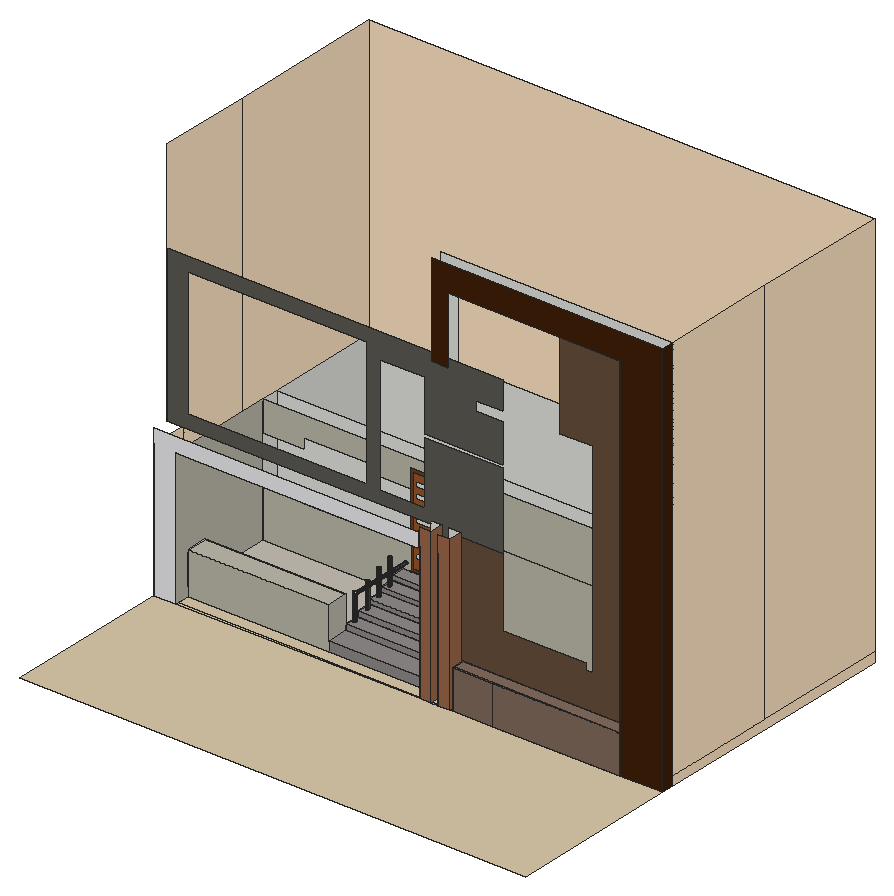
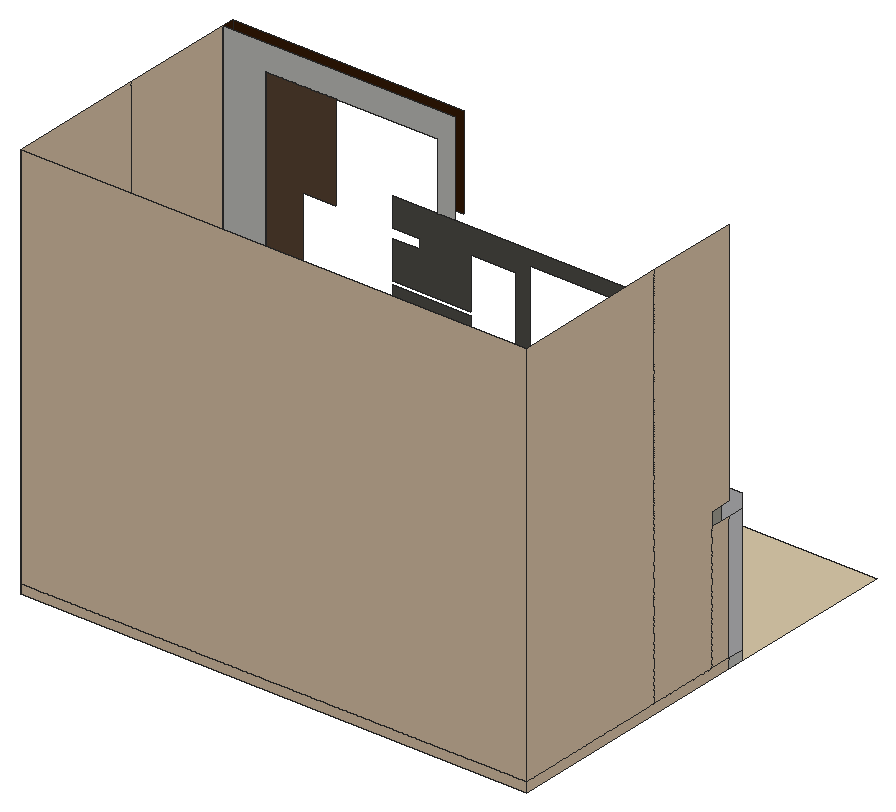
# SketchUp Ruby script. Lengths in inches.
U = 1.inch
M = Sketchup.active_model
def pt(a) = Geom::Point3d.new(a.map { |v| v * U })
def face(e, loops, mat)
  f = e.add_face(loops[0].map { |a| pt(a) })
  loops[1..].each { |l| e.add_face(l.map { |a| pt(a) }).erase! }
  f.material = f.back_material = mat if mat
  f
end
# faces: each face lists its corners as indices into pts; further lists are holes
def faces(e, pts, list, mat = nil) = list.each { |f| face(e, (f[0].is_a?(Array) ? f : [f]).map { |l| l.map { |i| pts[i] } }, mat) }
# xy, xz, yz: faces in a plane at the given z, y or x. An outline is a flat list of corners, or four numbers for a rectangle; further outlines are holes
def ring(l) = l.size == 4 ? [[l[0], l[1]], [l[2], l[1]], [l[2], l[3]], [l[0], l[3]]] : l.each_slice(2).to_a
def flat(e, list, mat, &to3) = list.each { |f| face(e, (f[0].is_a?(Array) ? f : [f]).map { |l| ring(l).map { |u, v| to3.(u, v) } }, mat) }
def xy(e, z, list, mat = nil) = flat(e, list, mat) { |x, y| [x, y, z] }
def xz(e, y, list, mat = nil) = flat(e, list, mat) { |x, z| [x, y, z] }
def yz(e, x, list, mat = nil) = flat(e, list, mat) { |y, z| [x, y, z] }
def lines(e, pts, list) = list.each { |a, b| e.add_line(pt(pts[a]), pt(pts[b])) }
# prism: a flat outline (further loops are holes) pulled along v
def prism(e, loops, v, mat = nil)
  f = face(e, loops, mat); d = Geom::Vector3d.new(v.map { |x| x * U })
  f.pushpull(f.normal.samedirection?(d) ? d.length : -d.length)
end
def box(e, o, s, mat = nil) = prism(e, [[o, [o[0] + s[0], o[1], o[2]], [o[0] + s[0], o[1] + s[1], o[2]], [o[0], o[1] + s[1], o[2]]]], [0, 0, s[2]], mat)
def at(x, y, z, deg = 0) = Geom::Transformation.translation(pt([x, y, z])) * Geom::Transformation.rotation(ORIGIN, Z_AXIS, deg.degrees)
def axes(o, x, y, z) = Geom::Transformation.new([*x, 0, *y, 0, *z, 0, *pt(o).to_a, 1])
def part(name) = M.definitions.add(name)
# library, detail: a bought-in or finely detailed component or shape, given as its bounding box
def library(name, o, s) = part(name).tap { |d| box(d.entities, o, s) }
def detail(e, o, s) = box(e.add_group.entities, o, s)
def put(e, d, t, mat = nil) = e.add_instance(d, t).tap { |i| i.material = mat if mat }
def group(e, t, mat = nil) = e.add_group.tap { |g| g.transformation = t; g.material = mat if mat }.entities
root = M.entities
M.materials.add("[0012_Bisque]").color = [255, 228, 196]
M.materials.add("[0043_SaddleBrown]").color = [63, 31, 8]
M.materials.add("[Blinds Vertical Pattern]").color = [237, 237, 239]
M.materials.add("[Cladding Siding Tan]").color = [102, 79, 59]
M.materials.add("[Field Rectangle Tile]").color = [196, 189, 179]
M.materials.add("[Field Square Tile]").color = [217, 201, 169]
M.materials.add("[Formica Graystone]").color = [91, 89, 83]
M.materials.add("[Formica Graystone]1").color = [188, 184, 170]
M.materials.add("[Granite Brown]").color = [130, 107, 93]
M.materials.add("[Quartz Light Grey]").color = [251, 251, 252]
M.materials.add("[Stone Marble]").color = [143, 138, 136]
M.materials.add("[Wood Cherry Original]").color = [152, 86, 42]
M.materials.add("[Wood Veneer 01]").color = [107, 62, 33]
M.materials.add("[Wood Veneer 01]1").color = [120, 70, 37]
M.materials.add("[Wood Veneer 02]").color = [155, 104, 74]
xy(root,0,[[0,159.45,20.26,162.83],[250.29,161.27,261.4375,162.83],[267.85,161.27,267.85,162.83,279,162.83,279,161.35],[267.85,161.27,279,161.35,279,161.27],[0,162.83,20.26,174.45],
  [250.29,162.83,261.4375,174.45],[267.85,162.83,279,174.45],[281.23,162.83,439.49,174.45],[439.49,162.83,480,174.45],[0,174.45,480,414.45]])
xy(root,0,[[0,0,0,159.45,20.26,159.45,250.29,161.14,250.29,161.27,261.4375,161.27,261.4375,161.22,267.85,161.27,279,161.27,279,161.35,319.23,161.65,439.49,162.53,480,162.83,480,0],[20.26,159.45,20.26,162.83,250.29,162.83,250.29,161.14],[261.4375,161.22,261.4375,162.83,267.85,162.83,267.85,161.27],[279,161.35,279,162.83,281.23,162.83,281.23,161.65,319.23,161.65],[20.26,162.83,250.29,174.45],
  [261.4375,162.83,267.85,174.45],[279,162.83,281.23,174.45]],"[Field Square Tile]")
xy(root,0,[[281.23,161.65,281.23,162.83,439.49,162.83,439.49,162.53,319.23,161.65],[439.49,162.53,439.49,162.83,480,162.83]],"[Quartz Light Grey]")
xy(root,9,[[439.49,174.45,459.74,194.72,459.74,283.36,480,283.36,480,174.45],[0,194.72,20.26,263.11],[153.32,194.72,250.29,208.86],[153.32,208.86,250.29,223],[153.32,223,250.29,236.75],
  [153.32,236.75,250.29,249.88],[153.32,249.88,250.29,263.11],[0,263.11,0,414.45,480,414.45,480,283.36,459.74,283.36,459.74,394.19,20.26,394.19,20.26,263.11],[20.26,263.11,459.74,279.66],[20.26,279.66,459.74,394.19]])
xy(root,9,[[20.26,194.72,153.32,263.11],[250.29,194.72,459.74,263.11]],"[Field Rectangle Tile]")
xy(root,9,[[153.32,174.45,250.29,194.72]],"[Stone Marble]")
xy(root,14.375,[[156.2,200.96,155.83,201.01,155.48,201.15,155.18,201.38,154.95,201.68,154.8125,202.03,154.76,202.4,154.8125,202.77,154.95,203.12,155.18,203.41,155.48,203.64,155.83,203.79,156.2,203.84,156.57,203.79,156.92,203.64,157.22,203.41,157.44,203.12,157.59,202.77,157.64,202.4,157.59,202.03,157.44,201.68,157.22,201.38,156.92,201.15,156.57,201.01]])
xy(root,14.375,[[[153.32,194.72,250.29,208.86],[156.2,200.96,155.83,201.01,155.48,201.15,155.18,201.38,154.95,201.68,154.8125,202.03,154.76,202.4,154.8125,202.77,154.95,203.12,155.18,203.41,155.48,203.64,155.83,203.79,156.2,203.84,156.57,203.79,156.92,203.64,157.22,203.41,157.44,203.12,157.59,202.77,157.64,202.4,157.59,202.03,157.44,201.68,157.22,201.38,156.92,201.15,156.57,201.01]]],"[Stone Marble]")
xy(root,19.125,[[157.37,214.23,157,214.28,156.65,214.43,156.35,214.66,156.125,214.95,155.98,215.3,155.93,215.67,155.98,216.04,156.125,216.39,156.35,216.6875,156.65,216.92,157,217.0625,157.37,217.11,157.74,217.0625,158.09,216.92,158.39,216.6875,158.62,216.39,158.76,216.04,158.81,215.67,158.76,215.3,158.62,214.95,158.39,214.66,158.09,214.43,157.74,214.28]])
xy(root,19.125,[[[153.32,208.86,250.29,223],[157.37,214.23,157,214.28,156.65,214.43,156.35,214.66,156.125,214.95,155.98,215.3,155.93,215.67,155.98,216.04,156.125,216.39,156.35,216.6875,156.65,216.92,157,217.0625,157.37,217.11,157.74,217.0625,158.09,216.92,158.39,216.6875,158.62,216.39,158.76,216.04,158.81,215.67,158.76,215.3,158.62,214.95,158.39,214.66,158.09,214.43,157.74,214.28]]],"[Stone Marble]")
xy(root,23.5,[[156.56,228.62,156.1875,228.66,155.84,228.81,155.54,229.04,155.3125,229.33,155.17,229.68,155.12,230.05,155.17,230.43,155.3125,230.77,155.54,231.07,155.84,231.3,156.1875,231.44,156.56,231.49,156.93,231.44,157.28,231.3,157.57,231.07,157.8,230.77,157.95,230.43,158,230.05,157.95,229.68,157.8,229.33,157.57,229.04,157.28,228.81,156.93,228.66]])
xy(root,23.5,[[[153.32,223,250.29,236.75],[156.56,228.62,156.1875,228.66,155.84,228.81,155.54,229.04,155.3125,229.33,155.17,229.68,155.12,230.05,155.17,230.43,155.3125,230.77,155.54,231.07,155.84,231.3,156.1875,231.44,156.56,231.49,156.93,231.44,157.28,231.3,157.57,231.07,157.8,230.77,157.95,230.43,158,230.05,157.95,229.68,157.8,229.33,157.57,229.04,157.28,228.81,156.93,228.66]]],"[Stone Marble]")
xy(root,27.3125,[[157.29,241.24,156.92,241.29,156.57,241.43,156.27,241.66,156.04,241.96,155.9,242.31,155.85,242.68,155.9,243.05,156.04,243.4,156.27,243.7,156.57,243.92,156.92,244.07,157.29,244.12,157.66,244.07,158.01,243.92,158.3,243.7,158.53,243.4,158.68,243.05,158.72,242.68,158.68,242.31,158.53,241.96,158.3,241.66,158.01,241.43,157.66,241.29]])
xy(root,27.3125,[[[153.32,236.75,250.29,249.88],[157.29,241.24,156.92,241.29,156.57,241.43,156.27,241.66,156.04,241.96,155.9,242.31,155.85,242.68,155.9,243.05,156.04,243.4,156.27,243.7,156.57,243.92,156.92,244.07,157.29,244.12,157.66,244.07,158.01,243.92,158.3,243.7,158.53,243.4,158.68,243.05,158.72,242.68,158.68,242.31,158.53,241.96,158.3,241.66,158.01,241.43,157.66,241.29]]],"[Stone Marble]")
xy(root,31.75,[[153.32,249.88,250.29,263.11]],"[Stone Marble]")
xy(root,36.58,[[281.23,161.65,319.23,161.65,439.49,162.53,439.49,162.83,281.23,162.83],[281.23,162.83,439.49,174.45]],"[Granite Brown]")
xy(root,38.75,[[156.2,200.96,155.83,201.01,155.48,201.15,155.18,201.38,154.95,201.68,154.8125,202.03,154.76,202.4,154.8125,202.77,154.95,203.12,155.18,203.41,155.48,203.64,155.83,203.79,156.2,203.84,156.57,203.79,156.92,203.64,157.22,203.41,157.44,203.12,157.59,202.77,157.64,202.4,157.59,202.03,157.44,201.68,157.22,201.38,156.92,201.15,156.57,201.01]])
xy(root,39.75,[[156.2,200.96,156.57,201.01,156.92,201.15,157.22,201.38,157.44,201.68,157.59,202.03,157.64,202.4,157.59,202.77,157.44,203.12,157.22,203.41,156.92,203.64,156.57,203.79,156.2,203.84,155.83,203.79,155.48,203.64,155.18,203.41,154.95,203.12,154.8125,202.77,154.76,202.4,154.8125,202.03,154.95,201.68,155.18,201.38,155.48,201.15,155.83,201.01]])
xy(root,39.75,[[20.26,174.45,153.32,194.72]],"[Formica Graystone]1")
xz(root,159.45,[[0,0,20.26,0,20.26,129,250.29,129,250.29,142.5625,0,142.5625]],"[Blinds Vertical Pattern]")
xz(root,161.27,[[250.29,0,261.4375,145.3125],[267.85,0,279,145.3125]],"[Wood Veneer 02]")
xz(root,161.65,[[281.23,0,319.23,36.58]],"[Granite Brown]")
xz(root,162.83,[[439.49,0,480,0,480,377.375,260.36,377.375,260.36,289.4375,276.43,289.4375,276.43,352.96,439.49,352.96]],"[0043_SaddleBrown]")
xz(root,174.45,[[250.29,0,261.4375,9],[267.85,0,279,9],[281.23,0,439.49,36.58],[439.49,0,480,9],[250.29,9,261.4375,145.3125],
  [439.49,9,439.49,352.96,276.43,352.96,276.43,289.4375,260.36,289.4375,260.36,377.375,480,377.375,480,9],[267.85,9,279,145.3125]])
xz(root,174.45,[[279,0,281.23,0,281.23,36.58,439.49,36.58,439.49,352.96,372.71,352.96,372.71,262.44,404.1,262.44,404.1,69.56,397.29,69.56,397.29,75.51,319.23,75.51,319.23,141.375,279,141.375]],"[Cladding Siding Tan]")
xz(root,174.45,[[261.4375,0,267.85,0,267.85,145.3125,279,145.3125,279,141.375,319.23,141.375,319.23,213.94,244.42,213.94,244.42,154.2,202.17,154.2,202.17,265.33,244.42,265.33,244.42,217.18,319.23,217.18,319.23,253.38,293.48,253.38,293.48,262.44,319.23,262.44,319.23,289.4375,0,289.4375,0,142.5625,189.35,142.5625,189.35,155,20.26,155,20.26,275.9375,189.35,275.9375,189.35,142.5625,250.29,142.5625,250.29,145.3125,261.4375,145.3125]],"[Formica Graystone]")
xz(root,174.45,[[20.26,0,153.32,39.75]],"[Formica Graystone]1")
xz(root,174.45,[[153.32,0,250.29,9]],"[Stone Marble]")
xz(root,194.72,[[20.26,9,153.32,39.75],[250.29,9,459.74,129]],"[Formica Graystone]1")
xz(root,194.72,[[153.32,9,250.29,14.375]],"[Stone Marble]")
xz(root,203.55,[[156.3,36.36,156.6,36.4,156.89,36.51,157.14,36.7,157.33,36.95,157.44,37.24,157.49,37.54,157.44,37.85,157.33,38.14,157.14,38.38,156.89,38.57,156.6,38.69,156.3,38.73,155.99,38.69,155.7,38.57,155.46,38.38,155.27,38.14,155.15,37.85,155.11,37.54,155.15,37.24,155.27,36.95,155.46,36.7,155.7,36.51,155.99,36.4]],"[Formica Graystone]")
xz(root,208.86,[[153.32,9,250.29,14.375]])
xz(root,208.86,[[153.32,14.375,250.29,19.125]],"[Stone Marble]")
xz(root,223,[[153.32,9,250.29,19.125]])
xz(root,223,[[153.32,19.125,250.29,23.5]],"[Stone Marble]")
xz(root,236.75,[[153.32,9,250.29,23.5]])
xz(root,236.75,[[153.32,23.5,250.29,27.3125]],"[Stone Marble]")
xz(root,249.88,[[153.32,9,250.29,27.3125]])
xz(root,249.88,[[153.32,27.3125,250.29,31.75]],"[Stone Marble]")
xz(root,263.11,[[153.32,9,250.29,31.75],[156.3,36.36,155.99,36.4,155.7,36.51,155.46,36.7,155.27,36.95,155.15,37.24,155.11,37.54,155.15,37.85,155.27,38.14,155.46,38.38,155.7,38.57,155.99,38.69,156.3,38.73,156.6,38.69,156.89,38.57,157.14,38.38,157.33,38.14,157.44,37.85,157.49,37.54,157.44,37.24,157.33,36.95,157.14,36.7,156.89,36.51,156.6,36.4]])
xz(root,263.11,[[250.29,9,459.74,9,459.74,129,20.26,129,20.26,100.02,58.93,100.02,58.93,109.5625,122.43,109.5625,122.43,102.34,161.07,102.34,161.07,119.5,219.13,119.5,219.13,31.75,250.29,31.75],[[20.26,9,153.32,9,153.32,31.75,161.07,31.75,161.07,58.93,122.43,58.93,122.43,53.75,58.93,53.75,58.93,57.76,20.26,57.76],[156.3,36.36,155.99,36.4,155.7,36.51,155.46,36.7,155.27,36.95,155.15,37.24,155.11,37.54,155.15,37.85,155.27,38.14,155.46,38.38,155.7,38.57,155.99,38.69,156.3,38.73,156.6,38.69,156.89,38.57,157.14,38.38,157.33,38.14,157.44,37.85,157.49,37.54,157.44,37.24,157.33,36.95,157.14,36.7,156.89,36.51,156.6,36.4]]],"[Formica Graystone]1")
xz(root,263.11,[[[163.89,34.57,189.63,34.57,189.63,69.82,186.95,69.82,186.95,89.25,189.63,89.25,189.63,116.6875,163.89,116.6875],[166.93,105.23,166.48,105.46,166.07,105.77,165.74,106.16,165.49,106.61,165.34,107.1,165.29,107.61,165.34,108.12,165.49,108.6,165.74,109.05,166.07,109.44,166.48,109.76,166.93,109.98,182.32,109.98,182.8,109.77,183.23,109.47,183.59,109.08,183.85,108.63,184.02,108.13,184.07,107.61,184.02,107.08,183.85,106.59,183.59,106.13,183.23,105.74,182.8,105.44,182.32,105.23],[166.93,94.98,166.48,95.21,166.07,95.52,165.74,95.91,165.49,96.36,165.34,96.85,165.29,97.36,165.34,97.87,165.49,98.35,165.74,98.8,166.07,99.19,166.48,99.51,166.93,99.73,182.32,99.73,182.8,99.52,183.23,99.22,183.59,98.83,183.85,98.38,184.02,97.88,184.07,97.36,184.02,96.83,183.85,96.34,183.59,95.88,183.23,95.49,182.8,95.19,182.32,94.98],[166.93,84.73,166.48,84.96,166.07,85.27,165.74,85.66,165.49,86.11,165.34,86.6,165.29,87.11,165.34,87.62,165.49,88.1,165.74,88.55,166.07,88.94,166.48,89.26,166.93,89.48,182.32,89.48,182.8,89.27,183.23,88.97,183.59,88.58,183.85,88.13,184.02,87.63,184.07,87.11,184.02,86.58,183.85,86.09,183.59,85.63,183.23,85.24,182.8,84.94,182.32,84.73],[166.93,74.48,166.48,74.71,166.07,75.02,165.74,75.41,165.49,75.86,165.34,76.35,165.29,76.86,165.34,77.37,165.49,77.85,165.74,78.3,166.07,78.69,166.48,79.01,166.93,79.23,182.32,79.23,182.8,79.02,183.23,78.72,183.59,78.33,183.85,77.88,184.02,77.38,184.07,76.86,184.02,76.33,183.85,75.84,183.59,75.38,183.23,74.99,182.8,74.69,182.32,74.48],[166.93,64.23,166.48,64.46,166.07,64.77,165.74,65.16,165.49,65.61,165.34,66.1,165.29,66.61,165.34,67.12,165.49,67.6,165.74,68.05,166.07,68.44,166.48,68.76,166.93,68.98,182.32,68.98,182.8,68.77,183.23,68.47,183.59,68.08,183.85,67.63,184.02,67.13,184.07,66.61,184.02,66.08,183.85,65.59,183.59,65.13,183.23,64.74,182.8,64.44,182.32,64.23],[166.93,53.98,166.48,54.21,166.07,54.52,165.74,54.91,165.49,55.36,165.34,55.85,165.29,56.36,165.34,56.87,165.49,57.35,165.74,57.8,166.07,58.19,166.48,58.51,166.93,58.73,182.32,58.73,182.8,58.52,183.23,58.22,183.59,57.83,183.85,57.38,184.02,56.88,184.07,56.36,184.02,55.83,183.85,55.34,183.59,54.88,183.23,54.49,182.8,54.19,182.32,53.98],[166.93,43.73,166.48,43.96,166.07,44.27,165.74,44.66,165.49,45.11,165.34,45.6,165.29,46.11,165.34,46.62,165.49,47.1,165.74,47.55,166.07,47.94,166.48,48.26,166.93,48.48,182.32,48.48,182.8,48.27,183.23,47.97,183.59,47.58,183.85,47.13,184.02,46.63,184.07,46.11,184.02,45.58,183.85,45.09,183.59,44.63,183.23,44.24,182.8,43.94,182.32,43.73]],[[191.9,34.57,216.32,34.57,216.32,116.6875,191.9,116.6875,191.9,89.19,194.09,89.19,194.09,69.69,191.9,69.69],[198.25,44.86,197.79,45.08,197.38,45.4,197.05,45.79,196.8,46.23,196.65,46.72,196.6,47.23,196.65,47.74,196.8,48.23,197.05,48.68,197.38,49.07,197.79,49.38,198.25,49.61,213.63,49.61,214.12,49.4,214.54,49.09,214.9,48.71,215.16,48.25,215.33,47.75,215.38,47.23,215.33,46.71,215.16,46.21,214.9,45.76,214.54,45.37,214.12,45.06,213.63,44.86],[198.25,54.92,197.79,55.15,197.38,55.46,197.05,55.85,196.8,56.3,196.65,56.79,196.6,57.29,196.65,57.8,196.8,58.29,197.05,58.74,197.38,59.13,197.79,59.44,198.25,59.67,213.63,59.67,214.12,59.46,214.54,59.16,214.9,58.77,215.16,58.32,215.33,57.82,215.38,57.29,215.33,56.77,215.16,56.27,214.9,55.82,214.54,55.43,214.12,55.13,213.63,54.92],[198.25,64.98,197.79,65.21,197.38,65.52,197.05,65.91,196.8,66.36,196.65,66.85,196.6,67.36,196.65,67.87,196.8,68.35,197.05,68.8,197.38,69.19,197.79,69.51,198.25,69.73,213.63,69.73,214.12,69.52,214.54,69.22,214.9,68.83,215.16,68.38,215.33,67.88,215.38,67.36,215.33,66.83,215.16,66.34,214.9,65.88,214.54,65.49,214.12,65.19,213.63,64.98],[198.25,75.04,197.79,75.27,197.38,75.59,197.05,75.97,196.8,76.42,196.65,76.91,196.6,77.42,196.65,77.93,196.8,78.42,197.05,78.86,197.38,79.25,197.79,79.57,198.25,79.79,213.63,79.79,214.12,79.59,214.54,79.28,214.9,78.89,215.16,78.44,215.33,77.94,215.38,77.42,215.33,76.9,215.16,76.4,214.9,75.94,214.54,75.56,214.12,75.25,213.63,75.04],[198.25,85.11,197.79,85.33,197.38,85.65,197.05,86.04,196.8,86.48,196.65,86.97,196.6,87.48,196.65,87.99,196.8,88.48,197.05,88.93,197.38,89.32,197.79,89.63,198.25,89.86,213.63,89.86,214.12,89.65,214.54,89.34,214.9,88.96,215.16,88.5,215.33,88,215.38,87.48,215.33,86.96,215.16,86.46,214.9,86.01,214.54,85.62,214.12,85.31,213.63,85.11],[198.25,95.17,197.79,95.4,197.38,95.71,197.05,96.1,196.8,96.55,196.65,97.04,196.6,97.54,196.65,98.05,196.8,98.54,197.05,98.99,197.38,99.38,197.79,99.69,198.25,99.92,213.63,99.92,214.12,99.71,214.54,99.41,214.9,99.02,215.16,98.57,215.33,98.07,215.38,97.54,215.33,97.02,215.16,96.52,214.9,96.07,214.54,95.68,214.12,95.38,213.63,95.17],[198.25,105.23,197.79,105.46,197.38,105.77,197.05,106.16,196.8,106.61,196.65,107.1,196.6,107.61,196.65,108.12,196.8,108.6,197.05,109.05,197.38,109.44,197.79,109.76,198.25,109.98,213.63,109.98,214.12,109.77,214.54,109.47,214.9,109.08,215.16,108.63,215.33,108.13,215.38,107.61,215.33,107.08,215.16,106.59,214.9,106.13,214.54,105.74,214.12,105.44,213.63,105.23]]],"[Wood Cherry Original]")
xz(root,263.11,[[[161.07,31.75,219.13,119.5],[163.89,34.57,216.32,116.6875]]],"[Wood Veneer 01]")
xz(root,263.11,[[189.63,34.57,191.9,116.6875]],"[Wood Veneer 01]1")
xz(root,279.66,[[20.26,9,459.74,129]])
xz(root,394.19,[[20.26,9,459.74,129]])
xz(root,414.45,[[0,0,480,9],[0,9,480,377.375]],"[0012_Bisque]")
yz(root,0,[[159.45,0,174.45,9]])
yz(root,0,[[174.45,0,414.45,9],[174.45,9,194.72,129],[194.72,9,194.72,142.5625,174.45,142.5625,174.45,377.375,263.11,377.375,263.11,9],[263.11,9,414.45,377.375]],"[0012_Bisque]")
yz(root,0,[[159.45,9,174.45,129]],"[Blinds Vertical Pattern]")
yz(root,20.26,[[174.45,9,194.72,39.75],[263.11,9,279.66,129],[279.66,9,394.19,129]])
yz(root,20.26,[[159.45,0,174.45,0,174.45,39.75,194.72,39.75,194.72,9,263.11,9,263.11,129,159.45,129]],"[Formica Graystone]1")
yz(root,153.32,[[174.45,9,194.72,39.75]],"[Formica Graystone]1")
yz(root,153.32,[[194.72,9,208.86,14.375],[208.86,9,223,19.125],[223,9,236.75,23.5],[236.75,9,249.88,27.3125],[249.88,9,263.11,31.75]],"[Stone Marble]")
yz(root,250.29,[[194.72,9,208.86,14.375]])
yz(root,250.29,[[174.45,9,194.72,129]],"[Formica Graystone]1")
yz(root,250.29,[[208.86,9,223,19.125],[223,9,236.75,23.5],[236.75,9,249.88,27.3125],[249.88,9,263.11,31.75]],"[Stone Marble]")
yz(root,250.29,[[161.27,0,174.45,129]],"[Wood Veneer 02]")
yz(root,261.4375,[[161.27,0,174.45,145.3125]],"[Wood Veneer 02]")
yz(root,267.85,[[161.27,0,174.45,129]],"[Wood Veneer 02]")
yz(root,279,[[161.27,0,174.45,145.3125]],"[Wood Veneer 02]")
yz(root,281.23,[[161.65,0,174.45,36.58]],"[Granite Brown]")
yz(root,439.49,[[162.83,0,174.45,9],[162.83,9,174.45,36.58]])
yz(root,439.49,[[162.83,36.58,174.45,352.96]],"[0043_SaddleBrown]")
yz(root,439.49,[[162.53,0,162.83,36.58]],"[Quartz Light Grey]")
yz(root,459.74,[[263.11,9,279.66,129],[279.66,9,283.36,129],[283.36,9,394.19,129]])
yz(root,459.74,[[194.72,9,263.11,129]],"[Formica Graystone]1")
yz(root,480,[[174.45,0,414.45,9],[174.45,9,283.36,377.375],[283.36,9,414.45,377.375]],"[0012_Bisque]")
yz(root,480,[[162.83,0,174.45,377.375]],"[0043_SaddleBrown]")
p = [[319.23,161.65,0],[439.49,162.53,0],[439.49,162.53,36.58],[319.23,161.65,36.58],[155.48,201.15,14.375],[155.83,201.01,14.375],
  [155.83,201.01,38.75],[155.48,201.15,38.75],[156.2,200.96,14.375],[156.2,200.96,38.75],[156.57,201.01,14.375],[156.57,201.01,38.75],
  [156.92,201.15,14.375],[156.92,201.15,38.75],[155.18,201.38,14.375],[155.18,201.38,38.75],[157.22,201.38,14.375],[157.22,201.38,38.75],
  [154.95,201.68,14.375],[154.95,201.68,38.75],[157.44,201.68,14.375],[157.44,201.68,38.75],[154.8125,202.03,14.375],[154.8125,202.03,38.75],
  [157.59,202.03,14.375],[157.59,202.03,38.75],[154.76,202.4,14.375],[154.76,202.4,38.75],[157.64,202.4,14.375],[157.64,202.4,38.75],
  [154.8125,202.77,14.375],[154.8125,202.77,38.75],[157.59,202.77,14.375],[157.59,202.77,38.75],[154.95,203.12,14.375],[154.95,203.12,38.75],
  [157.44,203.12,14.375],[157.44,203.12,38.75],[155.18,203.41,14.375],[155.18,203.41,38.75],[157.22,203.41,14.375],[157.22,203.41,38.75],
  [155.48,203.64,14.375],[155.48,203.64,38.75],[156.92,203.64,14.375],[156.92,203.64,38.75],[155.83,203.79,14.375],[155.83,203.79,38.75],
  [156.57,203.79,14.375],[156.57,203.79,38.75],[156.2,203.84,14.375],[156.2,203.84,38.75],[157,214.28,19.125],[157.37,214.23,19.125],
  [157.37,214.23,43.5],[157,214.28,43.5],[157.74,214.28,19.125],[157.74,214.28,43.5],[156.65,214.43,19.125],[156.65,214.43,43.5],
  [158.09,214.43,19.125],[158.09,214.43,43.5],[156.35,214.66,19.125],[156.35,214.66,43.5],[158.39,214.66,19.125],[158.39,214.66,43.5],
  [156.125,214.95,19.125],[156.125,214.95,43.5],[158.62,214.95,19.125],[158.62,214.95,43.5],[155.98,215.3,19.125],[155.98,215.3,43.5],
  [158.76,215.3,19.125],[158.76,215.3,43.5],[155.93,215.67,19.125],[155.93,215.67,43.5],[158.81,215.67,19.125],[158.81,215.67,43.5],
  [155.98,216.04,19.125],[155.98,216.04,43.5],[158.76,216.04,19.125],[158.76,216.04,43.5],[156.125,216.39,19.125],[156.125,216.39,43.5],
  [158.62,216.39,19.125],[158.62,216.39,43.5],[156.35,216.6875,19.125],[156.35,216.6875,43.5],[158.39,216.6875,19.125],[158.39,216.6875,43.5],
  [156.65,216.92,19.125],[156.65,216.92,43.5],[158.09,216.92,19.125],[158.09,216.92,43.5],[157,217.0625,19.125],[157,217.0625,43.5],
  [157.74,217.0625,19.125],[157.74,217.0625,43.5],[157.37,217.11,19.125],[157.37,217.11,43.5],[156.1875,228.66,23.5],[156.56,228.62,23.5],
  [156.56,228.62,47.875],[156.1875,228.66,47.875],[156.93,228.66,23.5],[156.93,228.66,47.875],[155.84,228.81,23.5],[155.84,228.81,47.875],
  [157.28,228.81,23.5],[157.28,228.81,47.875],[155.54,229.04,23.5],[155.54,229.04,47.875],[157.57,229.04,23.5],[157.57,229.04,47.875],
  [155.3125,229.33,23.5],[155.3125,229.33,47.875],[157.8,229.33,23.5],[157.8,229.33,47.875],[155.17,229.68,23.5],[155.17,229.68,47.875],
  [157.95,229.68,23.5],[157.95,229.68,47.875],[155.12,230.05,23.5],[155.12,230.05,47.875],[158,230.05,23.5],[158,230.05,47.875],
  [155.17,230.43,23.5],[155.17,230.43,47.875],[157.95,230.43,23.5],[157.95,230.43,47.875],[155.3125,230.77,23.5],[155.3125,230.77,47.875],
  [157.8,230.77,23.5],[157.8,230.77,47.875],[155.54,231.07,23.5],[155.54,231.07,47.875],[157.57,231.07,23.5],[157.57,231.07,47.875],
  [155.84,231.3,23.5],[155.84,231.3,47.875],[157.28,231.3,23.5],[157.28,231.3,47.875],[156.1875,231.44,23.5],[156.1875,231.44,47.875],
  [156.93,231.44,23.5],[156.93,231.44,47.875],[156.56,231.49,23.5],[156.56,231.49,47.875],[156.92,241.29,27.3125],[157.29,241.24,27.3125],
  [157.29,241.24,51.6875],[156.92,241.29,51.6875],[157.66,241.29,27.3125],[157.66,241.29,51.6875],[156.57,241.43,27.3125],[156.57,241.43,51.6875],
  [158.01,241.43,27.3125],[158.01,241.43,51.6875],[156.27,241.66,27.3125],[156.27,241.66,51.6875],[158.3,241.66,27.3125],[158.3,241.66,51.6875],
  [156.04,241.96,27.3125],[156.04,241.96,51.6875],[158.53,241.96,27.3125],[158.53,241.96,51.6875],[155.9,242.31,27.3125],[155.9,242.31,51.6875],
  [158.68,242.31,27.3125],[158.68,242.31,51.6875],[155.85,242.68,27.3125],[155.85,242.68,51.6875],[158.72,242.68,27.3125],[158.72,242.68,51.6875],
  [155.9,243.05,27.3125],[155.9,243.05,51.6875],[158.68,243.05,27.3125],[158.68,243.05,51.6875],[156.04,243.4,27.3125],[156.04,243.4,51.6875],
  [158.53,243.4,27.3125],[158.53,243.4,51.6875],[156.27,243.7,27.3125],[156.27,243.7,51.6875],[158.3,243.7,27.3125],[158.3,243.7,51.6875],
  [156.57,243.92,27.3125],[156.57,243.92,51.6875],[158.01,243.92,27.3125],[158.01,243.92,51.6875],[156.92,244.07,27.3125],[156.92,244.07,51.6875],
  [157.66,244.07,27.3125],[157.66,244.07,51.6875],[157.29,244.12,27.3125],[157.29,244.12,51.6875],[155.7,263.11,36.51],[155.99,263.11,36.4],
  [155.99,203.55,36.4],[155.7,203.55,36.51],[156.3,263.11,36.36],[156.3,203.55,36.36],[156.6,263.11,36.4],[156.6,203.55,36.4],
  [156.89,263.11,36.51],[156.89,203.55,36.51],[155.46,263.11,36.7],[155.46,203.55,36.7],[157.14,263.11,36.7],[157.14,203.55,36.7],
  [155.27,263.11,36.95],[155.27,203.55,36.95],[157.33,263.11,36.95],[157.33,203.55,36.95],[155.15,263.11,37.24],[155.15,203.55,37.24],
  [157.44,263.11,37.24],[157.44,203.55,37.24],[155.11,263.11,37.54],[155.11,203.55,37.54],[157.49,263.11,37.54],[157.49,203.55,37.54],
  [155.15,263.11,37.85],[155.15,203.55,37.85],[157.44,263.11,37.85],[157.44,203.55,37.85],[155.27,263.11,38.14],[155.27,203.55,38.14],
  [157.33,263.11,38.14],[157.33,203.55,38.14],[155.46,263.11,38.38],[155.46,203.55,38.38],[157.14,263.11,38.38],[157.14,203.55,38.38],
  [155.7,263.11,38.57],[155.7,203.55,38.57],[156.89,263.11,38.57],[156.89,203.55,38.57],[155.99,263.11,38.69],[155.99,203.55,38.69],
  [156.6,263.11,38.69],[156.6,203.55,38.69],[156.3,263.11,38.73],[156.3,203.55,38.73],[155.83,201.01,39.75],[155.48,201.15,39.75],
  [156.2,200.96,39.75],[156.57,201.01,39.75],[156.92,201.15,39.75],[155.18,201.38,39.75],[157.22,201.38,39.75],[154.95,201.68,39.75],
  [157.44,201.68,39.75],[154.8125,202.03,39.75],[157.59,202.03,39.75],[154.76,202.4,39.75],[157.64,202.4,39.75],[154.8125,202.77,39.75],
  [157.59,202.77,39.75],[154.95,203.12,39.75],[157.44,203.12,39.75],[155.18,203.41,39.75],[157.22,203.41,39.75],[155.48,203.64,39.75],
  [156.92,203.64,39.75],[155.83,203.79,39.75],[156.57,203.79,39.75],[156.2,203.84,39.75],[156.2,202.4,14.375],[156.2,202.4,38.75],
  [157.37,215.67,19.125],[157.37,215.67,43.5],[156.56,230.05,23.5],[156.56,230.05,47.875],[157.29,242.68,27.3125],[157.29,242.68,51.6875]]
faces(root,p,[[0,1,2,3]],"[Granite Brown]")
faces(root,p,[[4,5,6,7],[5,8,9,6],[8,10,11,9],[10,12,13,11],[14,4,7,15],[12,16,17,13],[18,14,15,19],[16,20,21,17],
  [22,18,19,23],[20,24,25,21],[26,22,23,27],[24,28,29,25],[30,26,27,31],[28,32,33,29],[34,30,31,35],[32,36,37,33],
  [38,34,35,39],[36,40,41,37],[42,38,39,43],[40,44,45,41],[46,42,43,47],[44,48,49,45],[50,46,47,51],[48,50,51,49],
  [52,53,54,55],[53,56,57,54],[58,52,55,59],[56,60,61,57],[62,58,59,63],[60,64,65,61],[66,62,63,67],[64,68,69,65],
  [70,66,67,71],[68,72,73,69],[74,70,71,75],[72,76,77,73],[78,74,75,79],[76,80,81,77],[82,78,79,83],[80,84,85,81],
  [86,82,83,87],[84,88,89,85],[90,86,87,91],[88,92,93,89],[94,90,91,95],[92,96,97,93],[98,94,95,99],[96,98,99,97],
  [100,101,102,103],[101,104,105,102],[106,100,103,107],[104,108,109,105],[110,106,107,111],[108,112,113,109],[114,110,111,115],[112,116,117,113],
  [118,114,115,119],[116,120,121,117],[122,118,119,123],[120,124,125,121],[126,122,123,127],[124,128,129,125],[130,126,127,131],[128,132,133,129],
  [134,130,131,135],[132,136,137,133],[138,134,135,139],[136,140,141,137],[142,138,139,143],[140,144,145,141],[146,142,143,147],[144,146,147,145],
  [148,149,150,151],[149,152,153,150],[154,148,151,155],[152,156,157,153],[158,154,155,159],[156,160,161,157],[162,158,159,163],[160,164,165,161],
  [166,162,163,167],[164,168,169,165],[170,166,167,171],[168,172,173,169],[174,170,171,175],[172,176,177,173],[178,174,175,179],[176,180,181,177],
  [182,178,179,183],[180,184,185,181],[186,182,183,187],[184,188,189,185],[190,186,187,191],[188,192,193,189],[194,190,191,195],[192,194,195,193],
  [196,197,198,199],[197,200,201,198],[200,202,203,201],[202,204,205,203],[206,196,199,207],[204,208,209,205],[210,206,207,211],[208,212,213,209],
  [214,210,211,215],[212,216,217,213],[218,214,215,219],[216,220,221,217],[222,218,219,223],[220,224,225,221],[226,222,223,227],[224,228,229,225],
  [230,226,227,231],[228,232,233,229],[234,230,231,235],[232,236,237,233],[238,234,235,239],[236,240,241,237],[242,238,239,243],[240,242,243,241]],"[Formica Graystone]")
faces(root,p,[[7,6,244,245],[6,9,246,244],[9,11,247,246],[11,13,248,247],[15,7,245,249],[13,17,250,248],[19,15,249,251],[17,21,252,250],
  [23,19,251,253],[21,25,254,252],[27,23,253,255],[25,29,256,254],[31,27,255,257],[29,33,258,256],[35,31,257,259],[33,37,260,258],
  [39,35,259,261],[37,41,262,260],[43,39,261,263],[41,45,264,262],[47,43,263,265],[45,49,266,264],[51,47,265,267],[49,51,267,266]])
lines(root,p,[[268,269],[270,271],[272,273],[274,275]])
